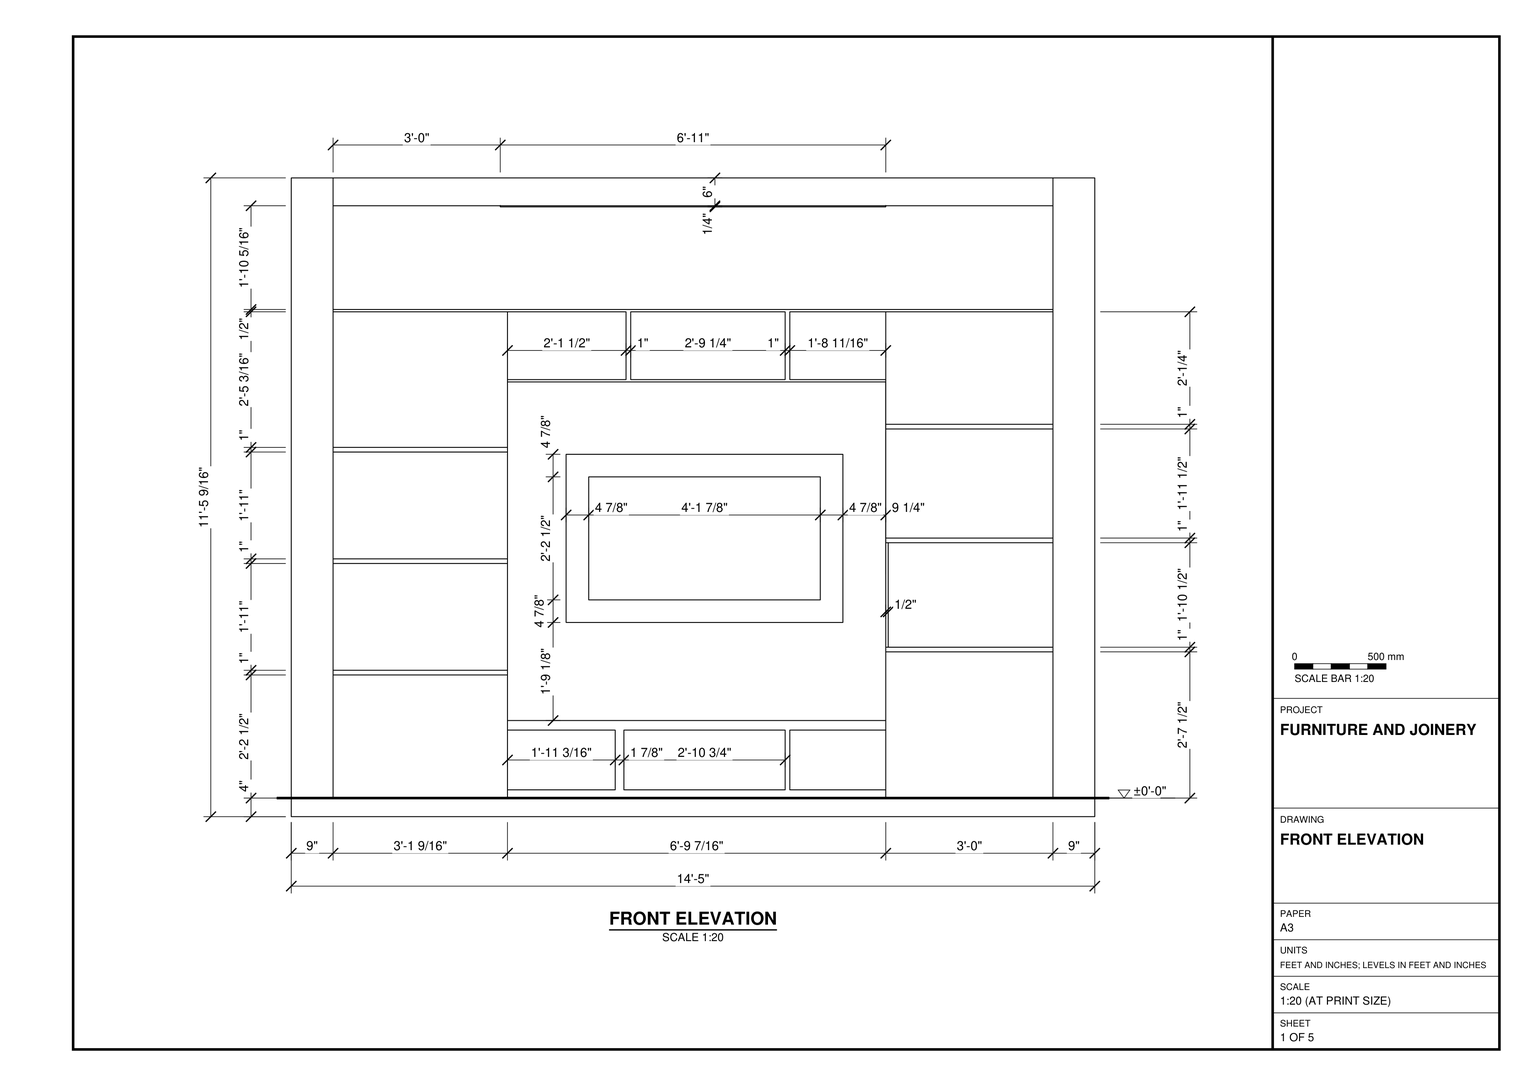
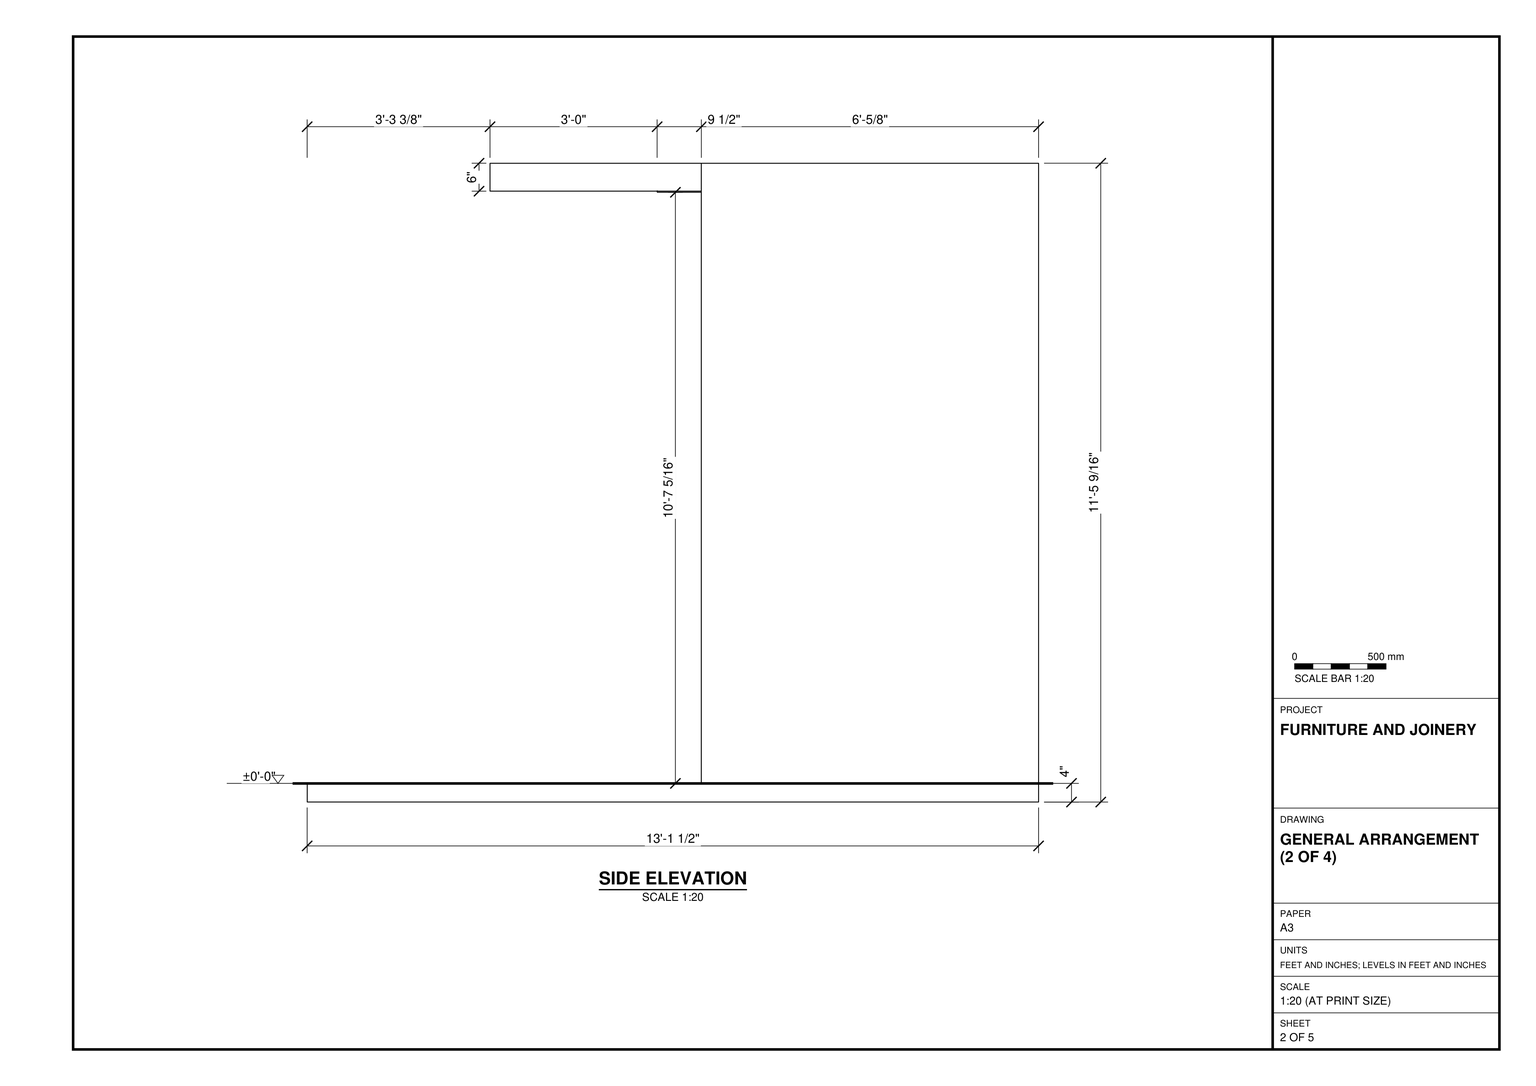
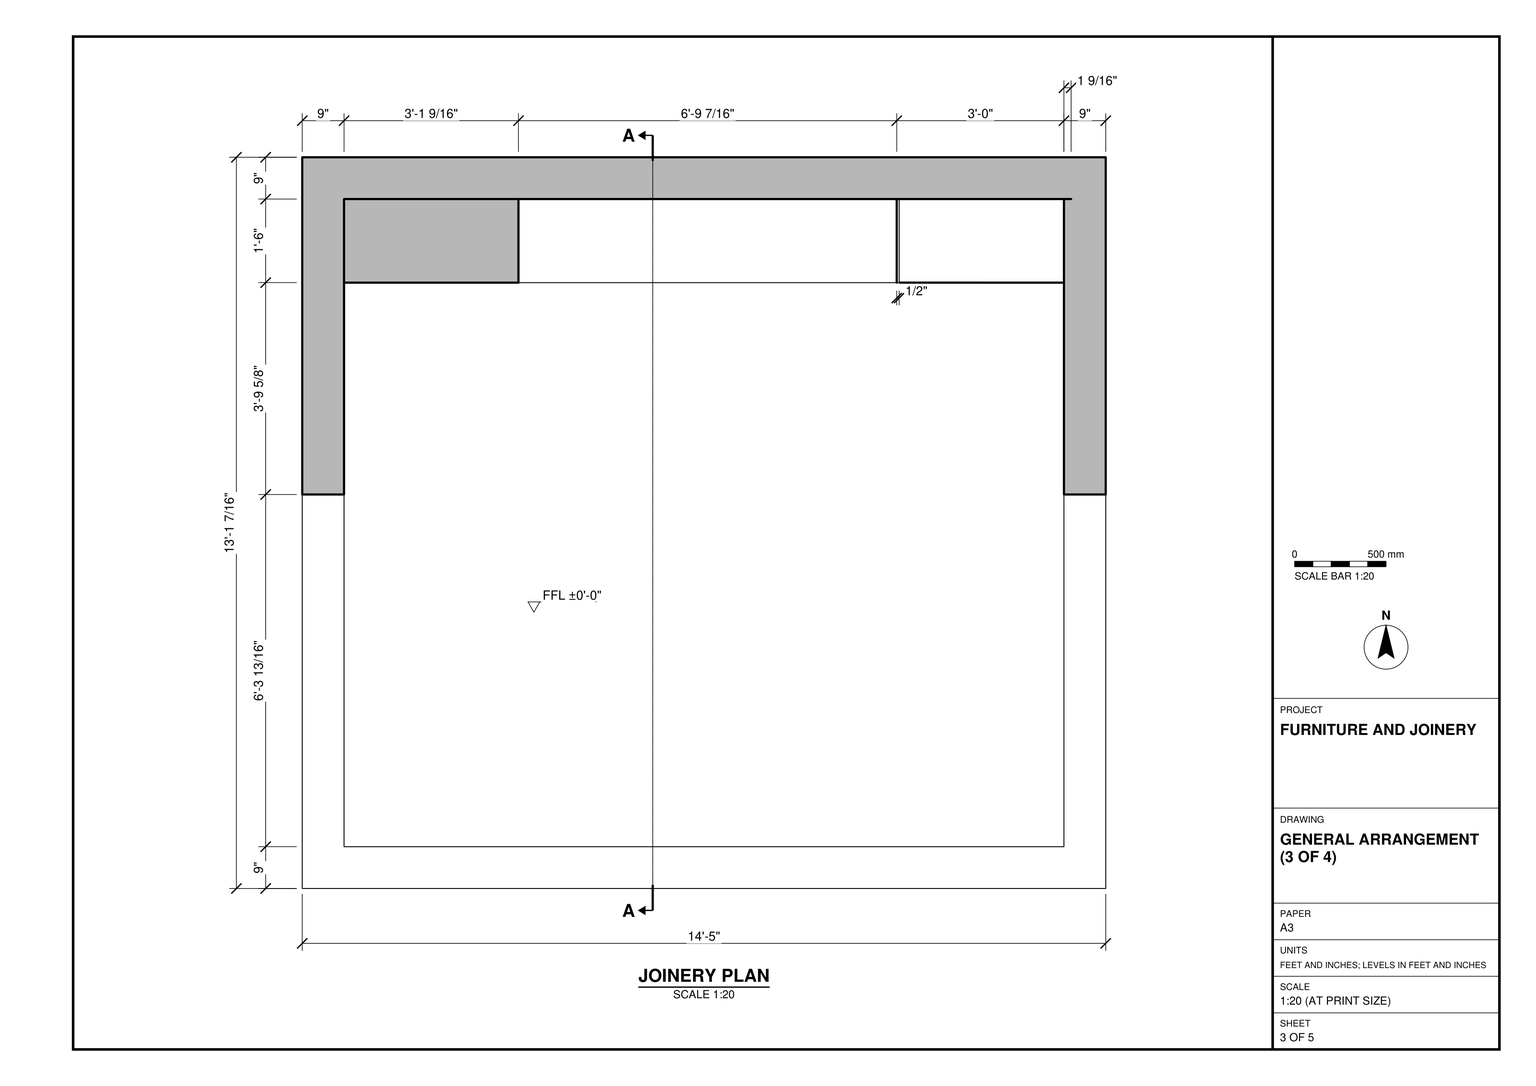
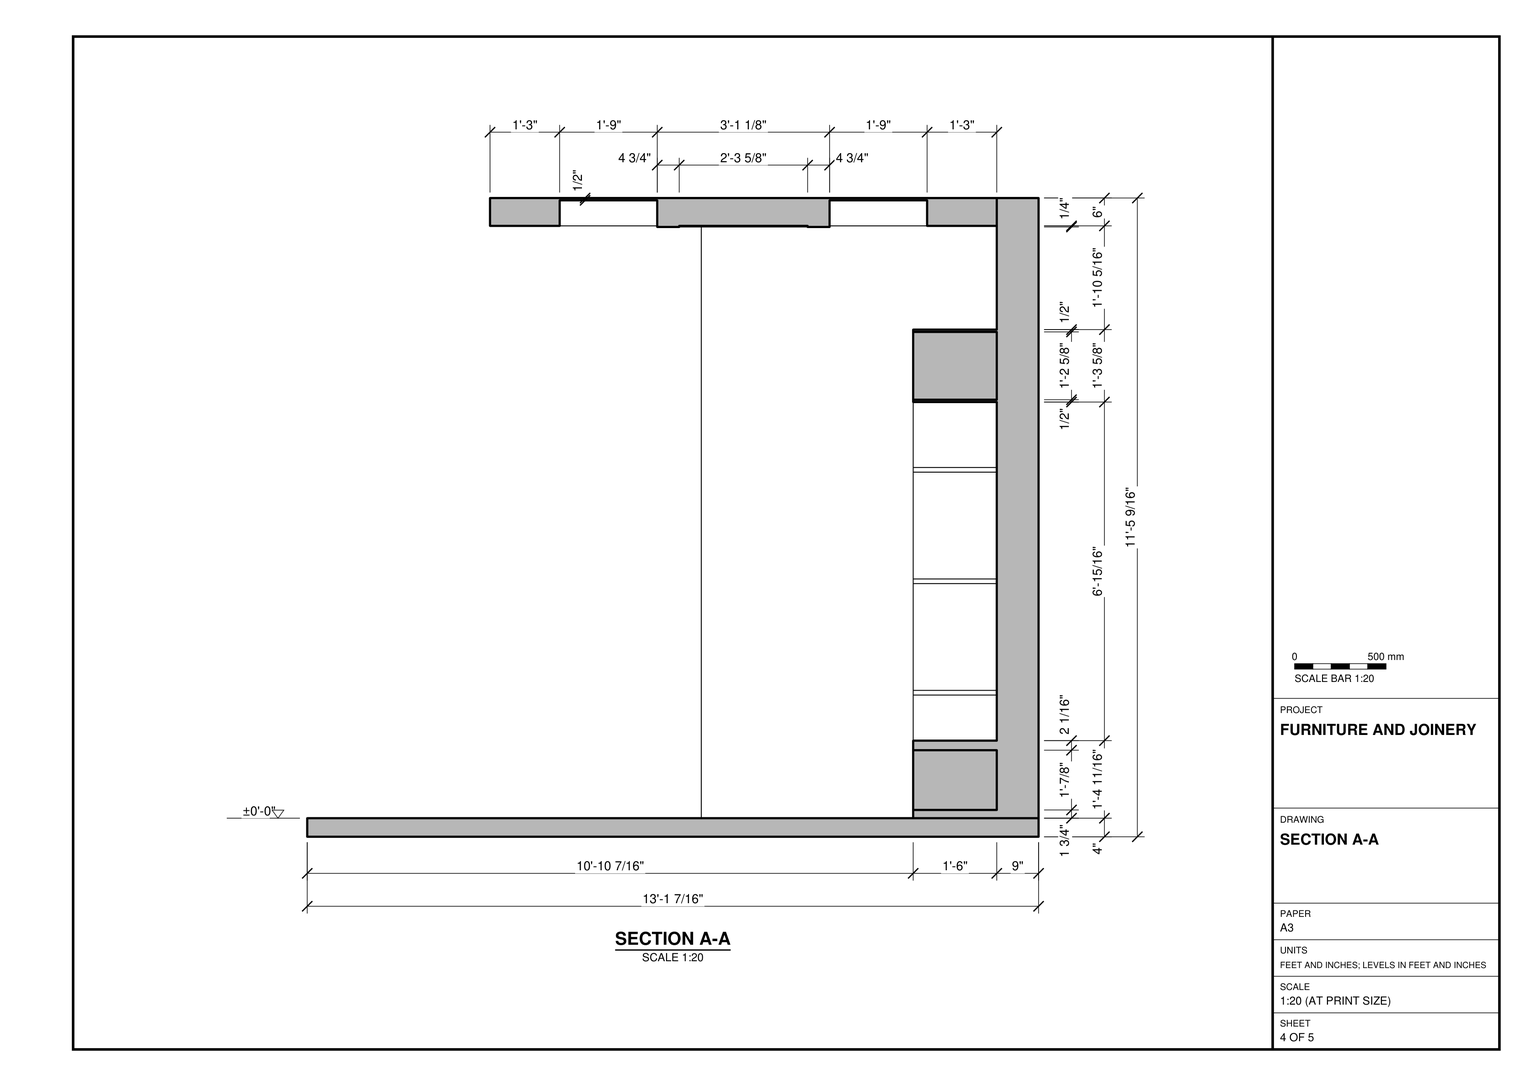
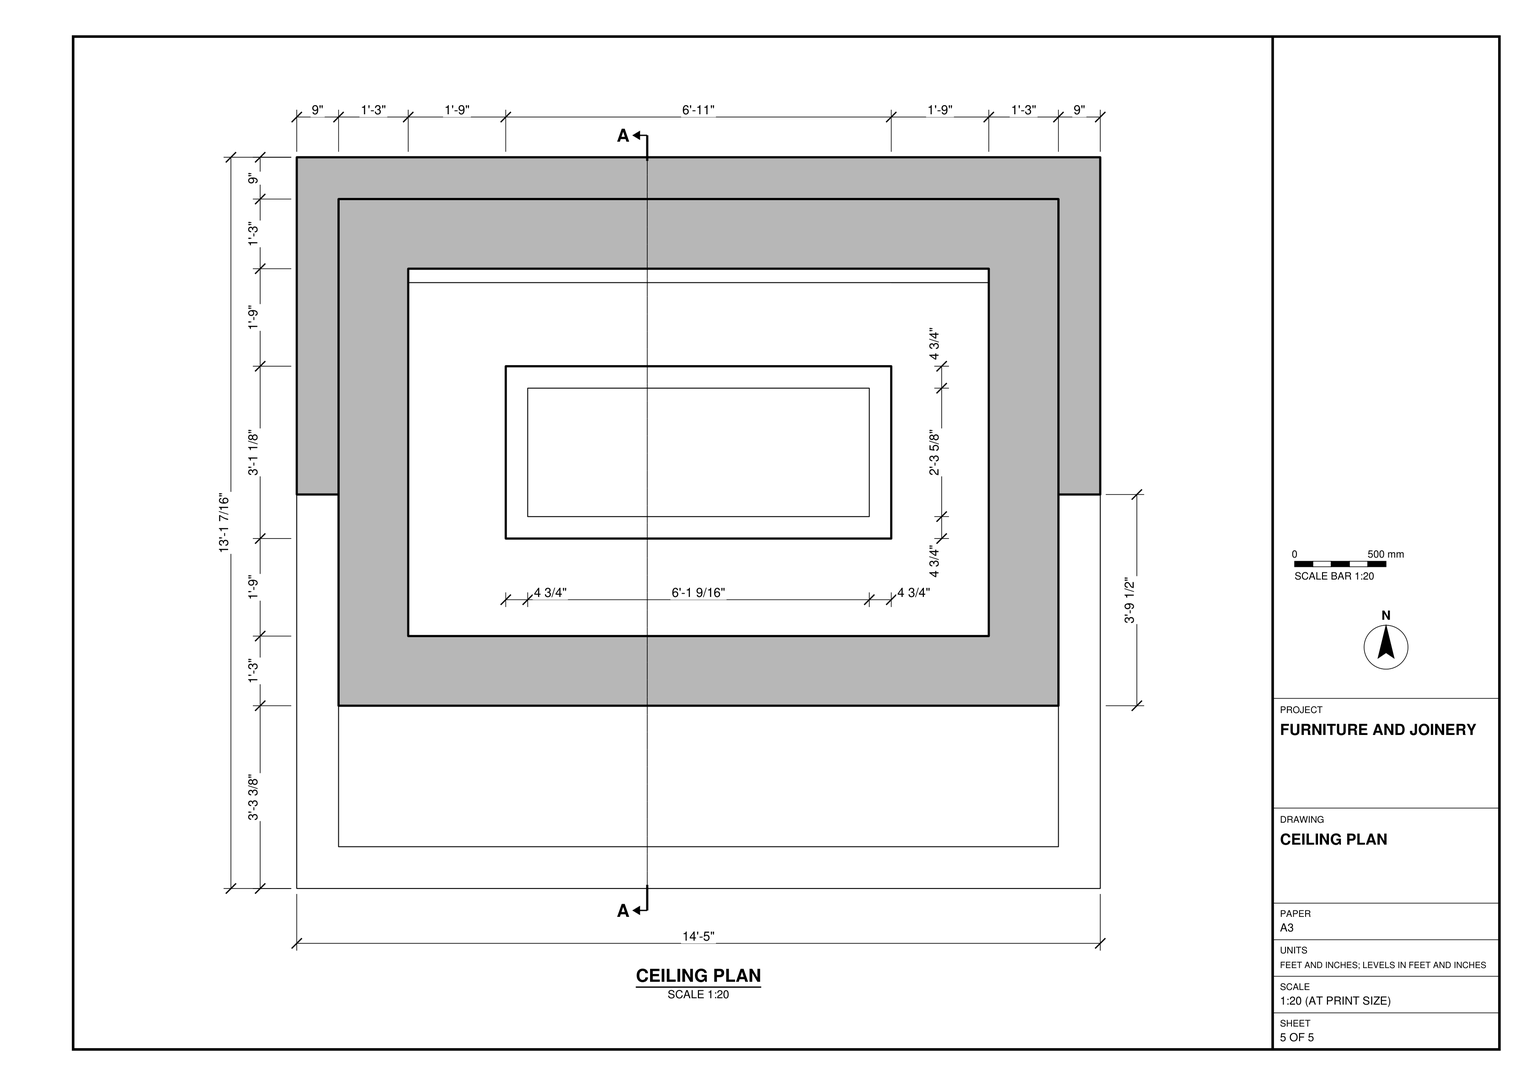
Build the display wall and its surrounding shell in SketchUp using task_files/diagram_01.pdf. Work in feet and inches. The overall model is 14'-5" wide, 13'-1 7/16" deep and 11'-5 9/16" high. Use ±0'-0" as the finished floor level, with the 4" floor slab below it.

Use the plan to set out the 9" back wall and side returns. Leave the front of the floor open. Follow the side elevation for the overhead slab: it projects beyond the side returns but stops short of the front floor edge. Fit the joinery against the back wall with a depth of 1'-6". In front elevation, set out the 3'-1 9/16" left shelving bay, the 6'-9 7/16" central display bay and the 3'-0" right shelving bay. Follow the shelf heights on each side rather than mirroring one bay onto the other. In the central bay, model the framed rectangular panel and the divided compartments above and below it. Use the dimensioned shelf and partition thicknesses so the clear openings match the elevation.

Keep shell elements and each joinery piece in separate groups or components, and use components for identical repeated parts. Decor and loose items, if used, may be any suitable library components. Save one SketchUp model as output_files/built_in_display_wall_with_flanking_shelves.skp.

# SketchUp Ruby script. Lengths in inches.
U = 1.inch
M = Sketchup.active_model
def pt(a) = Geom::Point3d.new(a.map { |v| v * U })
def face(e, loops, mat)
  f = e.add_face(loops[0].map { |a| pt(a) })
  loops[1..].each { |l| e.add_face(l.map { |a| pt(a) }).erase! }
  f.material = f.back_material = mat if mat
  f
end
# faces: each face lists its corners as indices into pts; further lists are holes
def faces(e, pts, list, mat = nil) = list.each { |f| face(e, (f[0].is_a?(Array) ? f : [f]).map { |l| l.map { |i| pts[i] } }, mat) }
# xy, xz, yz: faces in a plane at the given z, y or x. An outline is a flat list of corners, or four numbers for a rectangle; further outlines are holes
def ring(l) = l.size == 4 ? [[l[0], l[1]], [l[2], l[1]], [l[2], l[3]], [l[0], l[3]]] : l.each_slice(2).to_a
def flat(e, list, mat, &to3) = list.each { |f| face(e, (f[0].is_a?(Array) ? f : [f]).map { |l| ring(l).map { |u, v| to3.(u, v) } }, mat) }
def xy(e, z, list, mat = nil) = flat(e, list, mat) { |x, y| [x, y, z] }
def xz(e, y, list, mat = nil) = flat(e, list, mat) { |x, z| [x, y, z] }
def yz(e, x, list, mat = nil) = flat(e, list, mat) { |y, z| [x, y, z] }
def lines(e, pts, list) = list.each { |a, b| e.add_line(pt(pts[a]), pt(pts[b])) }
# prism: a flat outline (further loops are holes) pulled along v
def prism(e, loops, v, mat = nil)
  f = face(e, loops, mat); d = Geom::Vector3d.new(v.map { |x| x * U })
  f.pushpull(f.normal.samedirection?(d) ? d.length : -d.length)
end
def box(e, o, s, mat = nil) = prism(e, [[o, [o[0] + s[0], o[1], o[2]], [o[0] + s[0], o[1] + s[1], o[2]], [o[0], o[1] + s[1], o[2]]]], [0, 0, s[2]], mat)
def at(x, y, z, deg = 0) = Geom::Transformation.translation(pt([x, y, z])) * Geom::Transformation.rotation(ORIGIN, Z_AXIS, deg.degrees)
def axes(o, x, y, z) = Geom::Transformation.new([*x, 0, *y, 0, *z, 0, *pt(o).to_a, 1])
def part(name) = M.definitions.add(name)
# library, detail: a bought-in or finely detailed component or shape, given as its bounding box
def library(name, o, s) = part(name).tap { |d| box(d.entities, o, s) }
def detail(e, o, s) = box(e.add_group.entities, o, s)
def put(e, d, t, mat = nil) = e.add_instance(d, t).tap { |i| i.material = mat if mat }
def group(e, t, mat = nil) = e.add_group.tap { |g| g.transformation = t; g.material = mat if mat }.entities
root = M.entities
M.materials.add("Emissive").color = [255, 253, 43]
M.materials.add("Glass_Sky Reflection_01").color = [126, 138, 183]
M.materials["Glass_Sky Reflection_01"].alpha = 0.25
M.materials.add("Marble_01_1K").color = [230, 221, 211]
M.materials.add("Marble_06_1K").color = [165, 150, 147]
M.materials.add("Marble_07_1K").color = [36, 34, 36]
M.materials.add("Plywood_01_1K").color = [125, 96, 64]
M.materials.add("Plywood_08_1K").color = [202, 166, 113]
M.materials.add("Wood_Floor_12_1K").color = [92, 75, 65]
c1 = part("Group3\#1")
p = [[0,0,0],[0,0,-9.71],[-4.61,0,-9.71],[30.01,-1.43,0],[-30.01,-1.43,0],[30.01,1.43,0],
  [30.01,0,0],[-30.01,1.43,0],[4.61,0,-9.71],[-30.01,0,0],[0,0,-15.72]]
lines(c1.entities,p,[[0,1],[1,2],[3,4],[5,6],[7,5],[1,8],[9,0],[0,6],[8,10],[4,9],[6,3],[2,10],
  [9,7]])
c2 = part("Rectangle Light")
put(c2.entities,c1,at(0,0,0))
xy(root,4,[[0,0,173,0,173,84.84,164,84.84,164,9,9,9,9,84.84,0,84.84]])
xy(root,4,[[9,9,164,9,164,148.46,128,148.46,128,130.46,46.55,130.46,46.55,148.46,9,148.46]],"Marble_07_1K")
xy(root,5.77,[[46.55,130.46,69.75,148.46],[71.62,130.46,106.34,148.46],[107.34,130.46,128,148.46]])
xy(root,18.64,[[46.55,130.46,69.75,148.46],[71.62,130.46,106.34,148.46],[107.34,130.46,128,148.46]])
xy(root,20.7,[[46.55,130.46,128,148.46]])
xy(root,30.52,[[9,130.46,46.55,148.46]])
xy(root,31.52,[[9,130.46,46.55,148.46]])
xy(root,35.48,[[128,130.46,128.52,148.46],[128.52,130.46,164,148.46]])
xy(root,36.48,[[128,130.46,128.52,148.46],[128.52,130.46,164,130.46,128.52,130.48],[164,130.46,164,148.46,128.52,148.46,128.52,130.48]])
xy(root,54.52,[[9,130.46,46.55,148.46]])
xy(root,55.52,[[9,130.46,46.55,148.46]])
xy(root,58.98,[[128,130.48,128.52,148.46],[128.52,130.48,164,148.46]])
xy(root,59.98,[[128,130.48,128,148.46,127.98,148.46],[128,130.48,128.02,148.46],[128.02,130.48,128.52,148.46],[128.52,130.48,164,148.46]])
xy(root,78.52,[[9,130.46,46.55,148.46]])
xy(root,79.52,[[9,130.46,46.55,148.46]])
xy(root,83.48,[[127.98,130.46,127.98,148.46,128,148.46],[127.98,130.46,128,148.46,128.02,148.46,128.02,130.46],[128.02,130.46,128.02,148.46,164,148.46,164,130.48],[128.02,130.46,164,130.48,164,130.46]])
xy(root,84.48,[[127.98,130.46,164,148.46]])
xy(root,93.61,[[46.55,130.46,46.55,148.46,128,148.46,127.98,130.46],[127.98,130.46,128,148.46,128,130.46]],"Plywood_08_1K")
xy(root,94.11,[[46.55,130.46,72.08,148.46],[73.08,130.46,106.34,148.46],[107.34,130.46,128,148.46]])
xy(root,108.71,[[9,130.46,46.55,148.46],[46.55,130.46,72.08,148.46],[73.08,130.46,106.34,148.46],[107.34,130.46,128,148.46],[128,130.46,164,148.46]])
xy(root,109.21,[[9,130.46,164,148.46]])
xy(root,131.31,[[[45,75.36,128,112.46],[49.73,80.08,123.27,107.74]]])
xy(root,131.55,[[[9,39.36,164,148.46],[21,51.36,152,136.46]],[[21,51.36,152,136.46],[24,54.36,149,133.46]],[49.73,80.08,123.27,107.74]])
xy(root,137.05,[[[24,54.36,149,133.46],[45,75.36,128,112.46]]])
xy(root,137.55,[[9,39.36,164,148.46],[0,84.84,9,84.84,9,148.46,164,148.46,164,84.84,173,84.84,173,157.46,0,157.46]])
xz(root,39.36,[[9,131.55,164,137.55]])
xz(root,54.36,[[24,131.55,149,137.05]])
xz(root,75.36,[[45,131.31,128,137.05]])
xz(root,80.08,[[49.73,131.31,123.27,131.55]])
xz(root,84.84,[[0,4,9,137.55],[164,4,173,137.55]])
xz(root,107.74,[[49.73,131.31,123.27,131.55]],"Emissive")
xz(root,112.46,[[45,131.31,128,137.05]])
xz(root,130.46,[[[46.55,4,128,4,128,5.77,107.34,5.77,107.34,18.64,128,18.64,128,20.7,46.55,20.7,46.55,18.64,69.75,18.64,69.75,5.77,46.55,5.77],[71.62,5.77,106.34,18.64]],[9,30.52,46.55,31.52],[128,35.48,164,36.48],[9,54.52,46.55,55.52],[9,78.52,46.55,79.52],
  [127.98,83.48,164,84.48],[127.98,84.48,128,93.61],[[46.55,93.61,128,93.61,128,94.11,107.34,94.11,107.34,108.71,164,108.71,164,109.21,9,109.21,9,108.71,72.08,108.71,72.08,94.11,46.55,94.11],[73.08,94.11,106.34,108.71]]])
xz(root,130.46,[[9,31.52,46.55,54.52],[9,55.52,46.55,78.52],[9,79.52,46.55,108.71],[128,84.48,164,108.71],[46.55,94.11,72.08,108.71],
  [73.08,94.11,106.34,108.71],[107.34,94.11,128,108.71]],"Glass_Sky Reflection_01")
xz(root,130.46,[[46.55,5.77,69.75,18.64],[71.62,5.77,106.34,18.64],[107.34,5.77,128,18.64]],"Marble_01_1K")
xz(root,130.48,[[128,58.98,164,59.98]])
xz(root,133.46,[[24,131.55,149,137.05]],"Emissive")
xz(root,148.46,[[46.55,5.77,69.75,18.64],[71.62,5.77,106.34,18.64],[107.34,5.77,128,18.64],[9,31.52,46.55,54.52],[164,35.98,165.55,35.98,165.55,59.98,164.02,59.98,164.02,59.48,164,59.48],
  [128,36.48,128,59.98,127.98,59.98],[128,36.48,164,58.98],[9,55.52,46.55,78.52],[164,59.48,164.02,59.98],[127.98,59.98,128,59.98,127.98,82.8],
  [128,59.98,164,59.98,164,83.48,127.98,83.48,127.98,82.8],[164,60.48,164.02,83.98],[9,79.52,46.55,108.71],[127.98,83.48,128,84.48],[128,83.48,164,84.48],
  [164,83.98,164.02,85.21],[127.98,84.48,128,84.48,128,93.61],[128,84.48,164,108.71],[46.55,94.11,72.08,108.71],[73.08,94.11,106.34,108.71],
  [107.34,94.11,128,108.71],[9,109.21,164,131.55],[9,131.55,164,137.55]])
xz(root,148.46,[[[46.55,20.7,128,20.7,128,36.48,127.98,59.98,127.98,84.48,128,93.61,46.55,93.61],[59.18,41.81,118.77,78.03]]],"Marble_01_1K")
xz(root,148.46,[[9,4,46.55,30.52],[128,4,164,35.48]],"Marble_06_1K")
xz(root,148.46,[[64.04,46.68,113.9,73.16]],"Plywood_01_1K")
xz(root,148.46,[[[59.18,41.81,118.77,78.03],[64.04,46.68,113.9,73.16]]],"Wood_Floor_12_1K")
xz(root,157.46,[[0,4,173,137.55]])
yz(root,0,[[84.84,4,157.46,137.55]])
yz(root,9,[[84.84,4,148.46,4,148.46,30.52,130.46,30.52,130.46,109.21,148.46,109.21,148.46,131.55,84.84,131.55],[130.46,31.52,148.46,54.52],[130.46,55.52,148.46,78.52],[130.46,79.52,148.46,108.71],[39.36,131.55,84.84,137.55],
  [84.84,131.55,148.46,137.55]])
yz(root,24,[[54.36,131.55,84.84,137.05],[84.84,131.55,133.46,137.05]],"Emissive")
yz(root,45,[[75.36,131.31,84.84,137.05],[84.84,131.31,112.46,137.05]])
yz(root,46.55,[[130.46,4,148.46,5.77],[130.46,5.77,148.46,18.64],[130.46,18.64,148.46,20.7],[130.46,30.52,148.46,31.52],[130.46,54.52,148.46,55.52],
  [130.46,78.52,148.46,79.52],[130.46,93.61,148.46,94.11],[130.46,94.11,148.46,108.71]])
yz(root,46.55,[[130.46,20.7,148.46,30.52],[130.46,31.52,148.46,54.52],[130.46,55.52,148.46,78.52],[130.46,79.52,148.46,93.61]],"Plywood_08_1K")
yz(root,49.73,[[80.08,131.31,84.84,131.55],[84.84,131.31,107.74,131.55]])
yz(root,69.75,[[130.46,5.77,148.46,18.64]])
yz(root,71.62,[[130.46,5.77,148.46,18.64]])
yz(root,72.08,[[130.46,94.11,148.46,108.71]])
yz(root,73.08,[[130.46,94.11,148.46,108.71]])
yz(root,106.34,[[130.46,5.77,148.46,18.64],[130.46,94.11,148.46,108.71]])
yz(root,107.34,[[130.46,5.77,148.46,18.64],[130.46,94.11,148.46,108.71]])
yz(root,123.27,[[80.08,131.31,84.84,131.55]])
yz(root,123.27,[[84.84,131.31,107.74,131.55]],"Emissive")
yz(root,127.98,[[130.46,83.48,148.46,84.48]])
yz(root,128,[[130.46,4,148.46,5.77],[130.46,5.77,148.46,18.64],[130.46,18.64,148.46,20.7],[130.46,35.48,148.46,36.48],[130.48,58.98,148.46,59.98],
  [130.46,93.61,148.46,94.11],[130.46,94.11,148.46,108.71],[75.36,131.31,84.84,137.05],[84.84,131.31,112.46,137.05]])
yz(root,128,[[130.46,20.7,148.46,35.48],[130.46,36.48,148.46,58.98]],"Plywood_08_1K")
yz(root,149,[[54.36,131.55,84.84,137.05],[84.84,131.55,133.46,137.05]],"Emissive")
yz(root,164,[[84.84,4,84.84,131.55,148.46,131.55,148.46,109.21,130.46,109.21,130.46,108.71,148.46,108.71,148.46,83.48,130.48,83.48,130.48,59.98,148.46,59.98,148.46,35.98,130.46,35.98,130.46,35.48,148.46,35.48,148.46,4],[130.46,35.98,148.46,36.48],[130.48,58.98,148.46,59.48],[130.48,59.48,148.46,59.98],[130.48,59.98,148.46,83.48],
  [130.46,83.48,148.46,83.98],[130.46,83.98,148.46,84.48],[130.46,84.48,148.46,108.71],[39.36,131.55,84.84,137.55],[84.84,131.55,148.46,137.55]])
yz(root,173,[[84.84,4,157.46,137.55]])
p = [[164,130.46,58.98],[128.52,130.48,58.98],[128.52,130.48,36.48],[164,130.46,36.48],[164,130.48,83.48],[128.02,130.46,83.48],
  [128.02,130.46,59.98],[164,130.48,59.98],[127.98,148.46,59.98],[128,130.48,59.98],[128,130.48,84.48],[127.98,148.46,84.48],
  [127.98,148.46,83.48],[127.98,148.46,82.8],[128,148.46,84.48],[128,148.46,83.48],[127.98,130.46,83.48],[127.98,130.46,84.48],
  [127.98,130.46,93.61],[128,148.46,93.61],[128,148.46,4],[128,148.46,3.18],[164.5,148.46,83.98],[165.55,148.46,83.98],
  [128.5,148.96,83.98],[164,148.96,83.98],[127.98,148.96,83.98],[164.02,148.46,83.98]]
faces(root,p,[[0,1,2,3],[4,5,6,7]],"Glass_Sky Reflection_01")
faces(root,p,[[8,9,10,11,12,13],[14,15,16,17,18,19]],"Plywood_08_1K")
lines(root,p,[[20,21],[22,23],[24,25],[26,24],[27,22]])
put(root,c2,axes([88.94,148.45,81.35],[1,0,0],[0,0,-1],[0,1,0]))
g1 = group(root,at(0,0,0))
box(g1,[0,0,0],[173,157.46,4])
